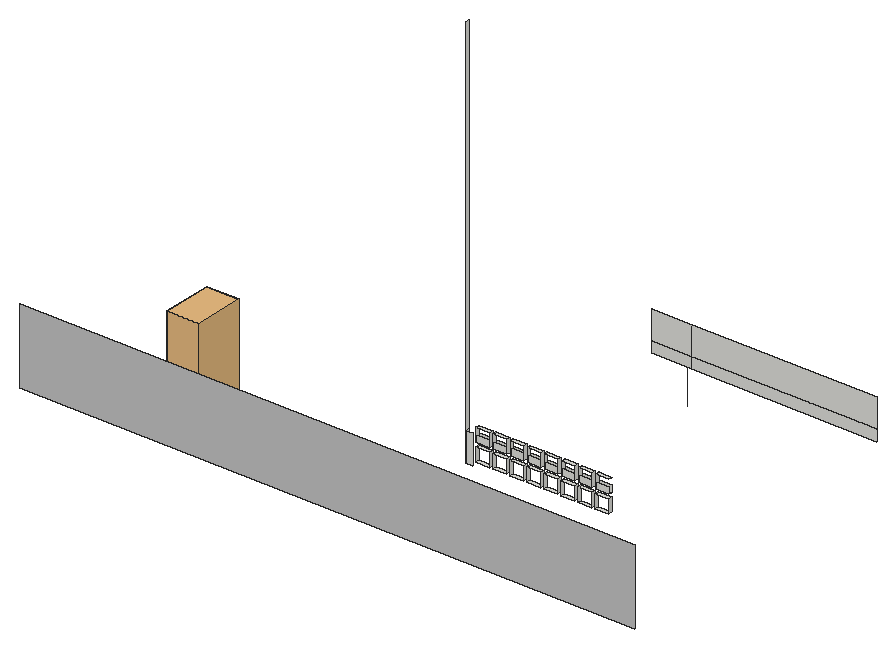
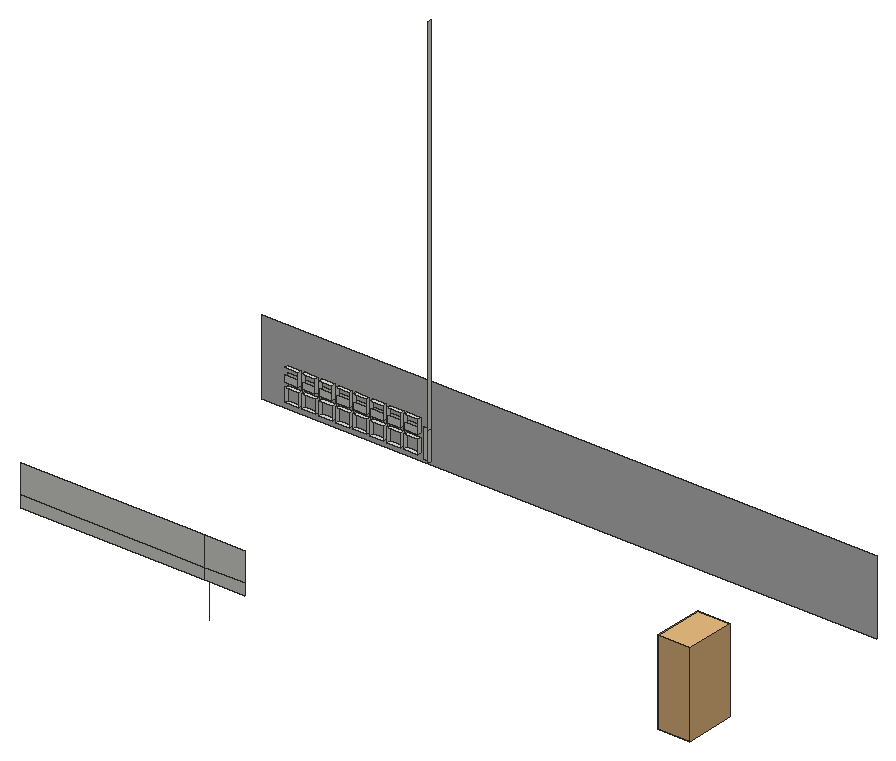
# SketchUp Ruby script. Lengths in inches.
U = 1.inch
M = Sketchup.active_model
def pt(a) = Geom::Point3d.new(a.map { |v| v * U })
def face(e, loops, mat)
  f = e.add_face(loops[0].map { |a| pt(a) })
  loops[1..].each { |l| e.add_face(l.map { |a| pt(a) }).erase! }
  f.material = f.back_material = mat if mat
  f
end
# faces: each face lists its corners as indices into pts; further lists are holes
def faces(e, pts, list, mat = nil) = list.each { |f| face(e, (f[0].is_a?(Array) ? f : [f]).map { |l| l.map { |i| pts[i] } }, mat) }
# xy, xz, yz: faces in a plane at the given z, y or x. An outline is a flat list of corners, or four numbers for a rectangle; further outlines are holes
def ring(l) = l.size == 4 ? [[l[0], l[1]], [l[2], l[1]], [l[2], l[3]], [l[0], l[3]]] : l.each_slice(2).to_a
def flat(e, list, mat, &to3) = list.each { |f| face(e, (f[0].is_a?(Array) ? f : [f]).map { |l| ring(l).map { |u, v| to3.(u, v) } }, mat) }
def xy(e, z, list, mat = nil) = flat(e, list, mat) { |x, y| [x, y, z] }
def xz(e, y, list, mat = nil) = flat(e, list, mat) { |x, z| [x, y, z] }
def yz(e, x, list, mat = nil) = flat(e, list, mat) { |y, z| [x, y, z] }
def lines(e, pts, list) = list.each { |a, b| e.add_line(pt(pts[a]), pt(pts[b])) }
# prism: a flat outline (further loops are holes) pulled along v
def prism(e, loops, v, mat = nil)
  f = face(e, loops, mat); d = Geom::Vector3d.new(v.map { |x| x * U })
  f.pushpull(f.normal.samedirection?(d) ? d.length : -d.length)
end
def box(e, o, s, mat = nil) = prism(e, [[o, [o[0] + s[0], o[1], o[2]], [o[0] + s[0], o[1] + s[1], o[2]], [o[0], o[1] + s[1], o[2]]]], [0, 0, s[2]], mat)
def at(x, y, z, deg = 0) = Geom::Transformation.translation(pt([x, y, z])) * Geom::Transformation.rotation(ORIGIN, Z_AXIS, deg.degrees)
def axes(o, x, y, z) = Geom::Transformation.new([*x, 0, *y, 0, *z, 0, *pt(o).to_a, 1])
def part(name) = M.definitions.add(name)
# library, detail: a bought-in or finely detailed component or shape, given as its bounding box
def library(name, o, s) = part(name).tap { |d| box(d.entities, o, s) }
def detail(e, o, s) = box(e.add_group.entities, o, s)
def put(e, d, t, mat = nil) = e.add_instance(d, t).tap { |i| i.material = mat if mat }
def group(e, t, mat = nil) = e.add_group.tap { |g| g.transformation = t; g.material = mat if mat }.entities
root = M.entities
M.materials.add("[Color M02]").color = [198, 198, 198]
c1 = library("Group\#13",[0,0,0],[3.54,3.54,3.9375])
xy(root,259.68,[[951.47,2332.13,953.78,2332.76],[954.38,2332.13,956.69,2332.76],[957.29,2332.13,959.6,2332.76],[960.2,2332.13,962.51,2332.76],[963.11,2332.13,965.43,2332.76],
  [966.03,2332.13,968.34,2332.76],[968.9375,2332.13,971.25,2332.76],[971.85,2332.13,974.16,2332.76]])
xy(root,262,[[951.47,2332.13,953.78,2332.76],[954.38,2332.13,956.69,2332.76],[957.29,2332.13,959.6,2332.76],[960.2,2332.13,962.51,2332.76],[963.11,2332.13,965.43,2332.76],
  [966.03,2332.13,968.34,2332.76],[968.9375,2332.13,971.25,2332.76],[971.85,2332.13,974.16,2332.76]])
xy(root,262.73,[[951.49,2332.13,953.81,2332.76],[954.41,2332.13,956.72,2332.76],[957.32,2332.13,959.63,2332.76],[960.23,2332.13,962.54,2332.76],[963.14,2332.13,965.46,2332.76],
  [966.06,2332.13,968.37,2332.76],[968.97,2332.13,971.28,2332.76],[971.88,2332.13,974.19,2332.76]])
xy(root,265.04,[[951.49,2332.13,953.81,2332.76],[954.41,2332.13,956.72,2332.76],[957.32,2332.13,959.63,2332.76],[960.23,2332.13,962.54,2332.76],[963.14,2332.13,965.46,2332.76],
  [966.06,2332.13,968.37,2332.76],[968.97,2332.13,971.28,2332.76],[971.88,2332.13,974.19,2332.76]])
xz(root,2321.87,[[881.75,251.0625,986.75,263.89]],"[Color M02]")
xz(root,2332.13,[[949.71,258.95,950.85,263.89],[951.49,262.73,953.81,263.89],[954.41,262.73,956.72,263.89],[957.32,262.73,959.63,263.89],[960.23,262.73,962.54,263.89],
  [963.14,262.73,965.46,263.89],[966.06,262.73,968.37,263.89],[968.97,262.73,971.28,263.89],[971.88,262.73,974.19,263.89]])
xz(root,2332.76,[[951.49,262.73,953.81,263.89],[954.41,262.73,956.72,263.89],[957.32,262.73,959.63,263.89],[960.23,262.73,962.54,263.89],[963.14,262.73,965.46,263.89],
  [966.06,262.73,968.37,263.89],[968.97,262.73,971.28,263.89],[971.88,262.73,974.19,263.89]])
xz(root,2373.56,[[948.3125,257.0625,955.23,258.95],[955.23,257.0625,986.75,258.95],[948.3125,258.95,955.23,263.89],[955.23,258.95,986.75,263.89]])
yz(root,949.71,[[2332.13,258.95,2332.76,263.89],[2332.13,263.89,2332.76,326.5]])
yz(root,951.47,[[2332.13,259.68,2332.76,262]])
yz(root,951.49,[[2332.13,262.73,2332.76,265.04]])
yz(root,953.78,[[2332.13,259.68,2332.76,262]])
yz(root,953.81,[[2332.13,262.73,2332.76,265.04]])
yz(root,954.38,[[2332.13,259.68,2332.76,262]])
yz(root,954.41,[[2332.13,262.73,2332.76,265.04]])
yz(root,956.69,[[2332.13,259.68,2332.76,262]])
yz(root,956.72,[[2332.13,262.73,2332.76,265.04]])
yz(root,957.29,[[2332.13,259.68,2332.76,262]])
yz(root,957.32,[[2332.13,262.73,2332.76,265.04]])
yz(root,959.6,[[2332.13,259.68,2332.76,262]])
yz(root,959.63,[[2332.13,262.73,2332.76,265.04]])
yz(root,960.2,[[2332.13,259.68,2332.76,262]])
yz(root,960.23,[[2332.13,262.73,2332.76,265.04]])
yz(root,962.51,[[2332.13,259.68,2332.76,262]])
yz(root,962.54,[[2332.13,262.73,2332.76,265.04]])
yz(root,963.11,[[2332.13,259.68,2332.76,262]])
yz(root,963.14,[[2332.13,262.73,2332.76,265.04]])
yz(root,965.43,[[2332.13,259.68,2332.76,262]])
yz(root,965.46,[[2332.13,262.73,2332.76,265.04]])
yz(root,966.03,[[2332.13,259.68,2332.76,262]])
yz(root,966.06,[[2332.13,262.73,2332.76,265.04]])
yz(root,968.34,[[2332.13,259.68,2332.76,262]])
yz(root,968.37,[[2332.13,262.73,2332.76,265.04]])
yz(root,968.9375,[[2332.13,259.68,2332.76,262]])
yz(root,968.97,[[2332.13,262.73,2332.76,265.04]])
yz(root,971.25,[[2332.13,259.68,2332.76,262]])
yz(root,971.28,[[2332.13,262.73,2332.76,265.04]])
yz(root,971.85,[[2332.13,259.68,2332.76,262]])
yz(root,971.88,[[2332.13,262.73,2332.76,265.04]])
yz(root,974.16,[[2332.13,259.68,2332.76,262]])
p = [[954.51,2373.56,251.0625],[954.51,2373.56,257.0625]]
lines(root,p,[[0,1]])
put(root,c1,axes([897.3,2340.62,258.17],[-1.5535,0,0],[0,2.39,0],[0,0,-3.63878]))
